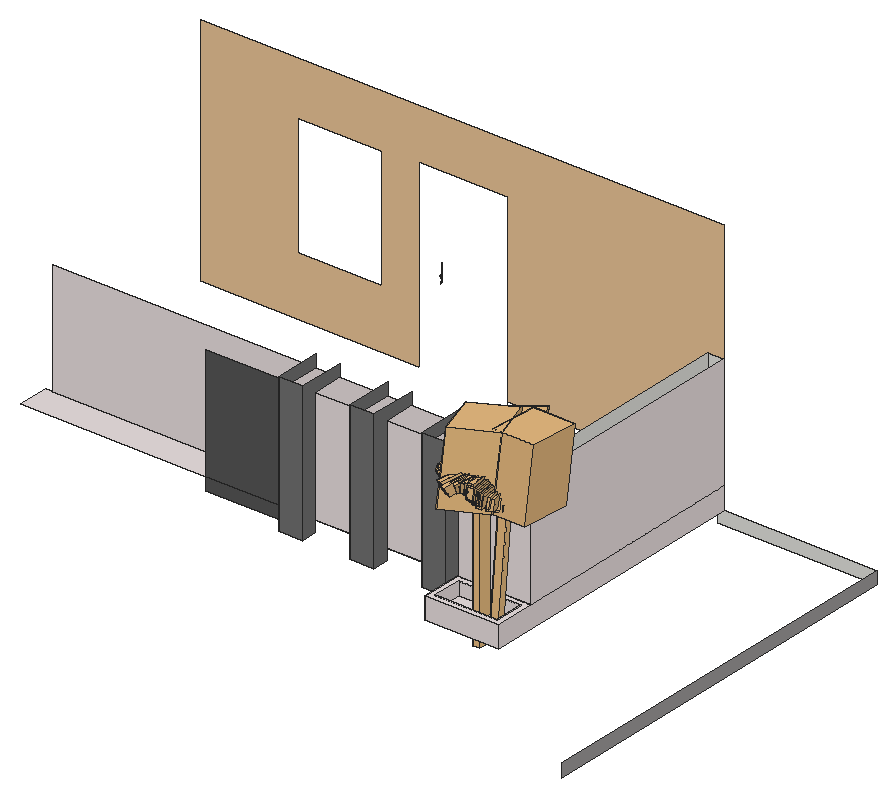
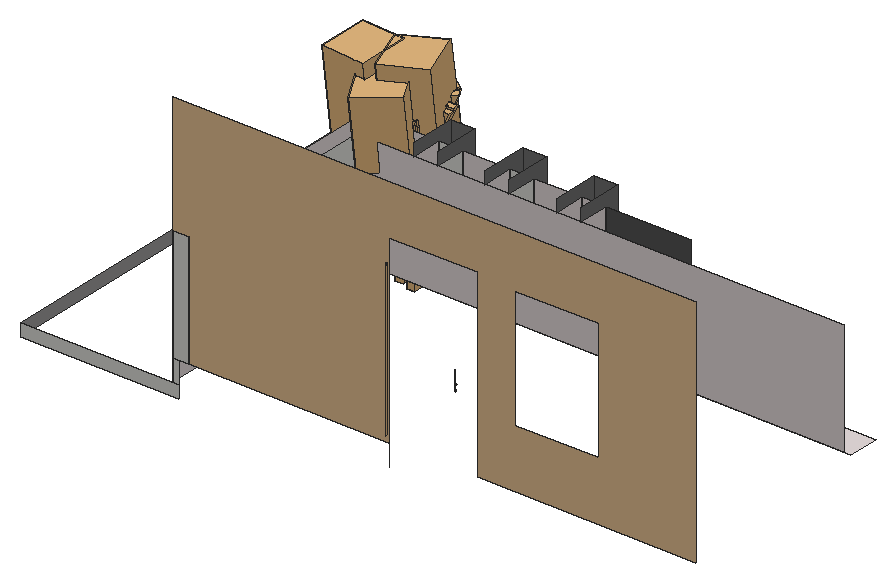
# SketchUp Ruby script. Lengths in inches.
U = 1.inch
M = Sketchup.active_model
def pt(a) = Geom::Point3d.new(a.map { |v| v * U })
def face(e, loops, mat)
  f = e.add_face(loops[0].map { |a| pt(a) })
  loops[1..].each { |l| e.add_face(l.map { |a| pt(a) }).erase! }
  f.material = f.back_material = mat if mat
  f
end
# faces: each face lists its corners as indices into pts; further lists are holes
def faces(e, pts, list, mat = nil) = list.each { |f| face(e, (f[0].is_a?(Array) ? f : [f]).map { |l| l.map { |i| pts[i] } }, mat) }
# xy, xz, yz: faces in a plane at the given z, y or x. An outline is a flat list of corners, or four numbers for a rectangle; further outlines are holes
def ring(l) = l.size == 4 ? [[l[0], l[1]], [l[2], l[1]], [l[2], l[3]], [l[0], l[3]]] : l.each_slice(2).to_a
def flat(e, list, mat, &to3) = list.each { |f| face(e, (f[0].is_a?(Array) ? f : [f]).map { |l| ring(l).map { |u, v| to3.(u, v) } }, mat) }
def xy(e, z, list, mat = nil) = flat(e, list, mat) { |x, y| [x, y, z] }
def xz(e, y, list, mat = nil) = flat(e, list, mat) { |x, z| [x, y, z] }
def yz(e, x, list, mat = nil) = flat(e, list, mat) { |y, z| [x, y, z] }
def lines(e, pts, list) = list.each { |a, b| e.add_line(pt(pts[a]), pt(pts[b])) }
# prism: a flat outline (further loops are holes) pulled along v
def prism(e, loops, v, mat = nil)
  f = face(e, loops, mat); d = Geom::Vector3d.new(v.map { |x| x * U })
  f.pushpull(f.normal.samedirection?(d) ? d.length : -d.length)
end
def box(e, o, s, mat = nil) = prism(e, [[o, [o[0] + s[0], o[1], o[2]], [o[0] + s[0], o[1] + s[1], o[2]], [o[0], o[1] + s[1], o[2]]]], [0, 0, s[2]], mat)
def at(x, y, z, deg = 0) = Geom::Transformation.translation(pt([x, y, z])) * Geom::Transformation.rotation(ORIGIN, Z_AXIS, deg.degrees)
def axes(o, x, y, z) = Geom::Transformation.new([*x, 0, *y, 0, *z, 0, *pt(o).to_a, 1])
def part(name) = M.definitions.add(name)
# library, detail: a bought-in or finely detailed component or shape, given as its bounding box
def library(name, o, s) = part(name).tap { |d| box(d.entities, o, s) }
def detail(e, o, s) = box(e.add_group.entities, o, s)
def put(e, d, t, mat = nil) = e.add_instance(d, t).tap { |i| i.material = mat if mat }
def group(e, t, mat = nil) = e.add_group.tap { |g| g.transformation = t; g.material = mat if mat }.entities
root = M.entities
M.materials.add("AM85_043_leaf").color = [102, 110, 36]
M.materials.add("AM85_043_stem").color = [137, 75, 57]
M.materials.add("Generic\#4").color = [113, 113, 113]
M.materials.add("Generic\#8").color = [235, 197, 151]
M.materials.add("Generic\#9").color = [233, 223, 223]
M.materials.add("Material \#1").color = [140, 140, 140]
M.materials.add("[Color M06]").color = [86, 86, 86]
M.materials.add("[Granite Dark Gray]").color = [158, 155, 155]
c1 = library("3DGeom~9_Defintion",[456.52,-471.89,-18.89],[5.57,1000,5.49])
c2 = library("3DGeom~7_Defintion",[455.56,-471.94,-18.85],[5.55,1000,5.48])
c3 = library("Group\#262",[721.75,-37.78,8.43],[46.9,73.44,671.88])
c4 = library("Group\#253",[26.16,5.88,-22.96],[170.57,196.24,312.95])
c5 = part("Leaf blade")
p = [[83.87,1.9,45.32],[93.74,4.15,37.73],[37.05,-3.5625,61.7],[49.38,-2.58,60.05],[69.4,9.27,54.68],[74.7,9.96,52.16],
  [102.49,6.87,29.18],[110.02,10.09,19.93],[45.83,5.6,61.35],[51.45,6.53,60.35],[91.18,12.19,41.53],[94.56,12.64,38.66],
  [12.82,-5.2,59.53],[24.77,-4.41,61.53],[22.59,0.63,61.46],[34.04,3.3,62.19],[61.47,-1.4,56.68],[73.04,0.08,51.71],
  [109.02,14.97,22.84],[115.89,16.47,11.9375]]
lines(c5.entities,p,[[0,1],[2,3],[4,5],[6,7],[8,9],[10,11],[12,13],[14,15],[16,17],[18,19]])
detail(c5.entities,[1.52,-6.02,0.37],[119.64,24.16,61.82])
c6 = part("Group\#250")
p = [[69.397,177.044,-76.908],[69.056,177.22,-76.772],[69.397,177.397,-76.635],[69.739,177.22,-76.772],[69.397,126.923,-36.489],[68.124,127.405,-35.832],
  [69.397,153.661,-55.129],[70.671,127.405,-35.832],[68.59,154.026,-54.756],[70.205,154.026,-54.756],[69.397,127.887,-35.175],[69.397,154.392,-54.384],
  [69.397,97.5,-21.509],[67.658,98.015,-20.533],[71.137,98.015,-20.533],[69.397,98.53,-19.558],[69.397,66.147,-10.6],[67.192,66.605,-9.289],
  [71.603,66.605,-9.289],[69.397,67.064,-7.977],[69.397,33.682,-4.048],[66.726,33.994,-2.4],[72.069,33.994,-2.4],[69.397,34.304,-0.752],
  [69.397,0.958,-2],[66.26,1.035,-0.035],[69.397,1.112,1.931],[72.535,1.035,-0.035],[69.397,0.956,-2]]
faces(c6.entities,p,[[0,1,2,3]])
faces(c6.entities,p,[[4,5,6],[4,6,7],[8,6,5],[9,7,6],[5,10,11,8],[7,9,11,10],[12,13,4],[12,4,14],
  [5,4,13],[7,14,4],[13,15,10,5],[14,7,10,15],[16,17,12],[16,12,18],[13,12,17],[14,18,12],
  [17,19,15,13],[18,14,15,19],[16,20,17],[16,18,20],[21,17,20],[22,20,18],[21,23,17],[22,18,23],
  [19,17,23],[19,23,18],[20,24,21],[20,22,24],[25,21,24],[25,26,21],[27,24,22],[22,23,27],
  [23,21,26],[28,25,24],[28,27,25],[28,24,27],[26,27,23],[26,25,27]],"AM85_043_stem")
c7 = library("Group\#264",[27.32,5.88,-22.96],[171.91,196.24,312.95])
c8 = library("Group\#274",[721.75,-37.78,8.43],[46.9,73.44,655.53])
xy(root,-6.625,[[458.275,57.753,489.122,72.622]],"Generic\#9")
xy(root,-6,[[408.209,67.75,420.146,75.375],[443.584,67.75,455.521,75.375]])
xy(root,-6,[[372.834,67.75,384.771,75.375]],"Generic\#9")
xy(root,0,[[[455.521,55,491.875,75.375],[458.275,57.753,489.122,72.622]],[238.793,75.375,491.875,75.375,491.875,194.8125,483.886,194.8125,483.886,90.9375,238.793,90.9375]],"Generic\#9")
xy(root,40.593,[[381.979,199.777,381.911,199.796,381.922,199.809],[381.979,199.777,381.922,199.809,381.983,199.793],[381.979,199.777,381.983,199.793,382.051,199.777],[382.051,199.777,381.983,199.793,382.047,199.793],[382.051,199.777,382.047,199.793,382.119,199.796],
  [382.047,199.793,382.108,199.809,382.119,199.796],[381.911,199.796,381.856,199.83,381.872,199.84],[381.911,199.796,381.872,199.84,381.922,199.809],[382.119,199.796,382.108,199.809,382.174,199.83],[382.108,199.809,382.158,199.84,382.174,199.83],
  [381.856,199.83,381.82,199.877,381.84,199.883],[381.856,199.83,381.84,199.883,381.872,199.84],[382.174,199.83,382.158,199.84,382.21,199.877],[382.158,199.84,382.19,199.883,382.21,199.877],[381.82,199.877,381.808,199.93,381.828,199.93],
  [381.82,199.877,381.828,199.93,381.84,199.883],[382.21,199.877,382.19,199.883,382.222,199.93],[382.19,199.883,382.201,199.93,382.222,199.93],[381.808,199.93,381.82,199.984,381.84,199.978],[381.808,199.93,381.84,199.978,381.828,199.93],
  [382.201,199.93,382.19,199.978,382.21,199.984],[382.201,199.93,382.21,199.984,382.222,199.93],[381.84,199.978,381.82,199.984,381.872,200.02],[382.19,199.978,382.158,200.02,382.174,200.03],[382.19,199.978,382.174,200.03,382.21,199.984],
  [381.82,199.984,381.856,200.03,381.872,200.02],[381.872,200.02,381.856,200.03,381.922,200.052],[382.158,200.02,382.108,200.052,382.119,200.065],[382.158,200.02,382.119,200.065,382.174,200.03],[381.856,200.03,381.911,200.065,381.922,200.052],
  [381.922,200.052,381.911,200.065,381.983,200.068],[382.108,200.052,382.047,200.068,382.051,200.084],[382.108,200.052,382.051,200.084,382.119,200.065],[381.911,200.065,381.979,200.084,381.983,200.068],[381.983,200.068,381.979,200.084,382.047,200.068],
  [382.047,200.068,381.979,200.084,382.051,200.084]],"Material \#1")
xy(root,40.61,[[381.979,199.777,381.983,199.793,381.911,199.796],[381.979,199.777,382.047,199.793,381.983,199.793],[381.979,199.777,382.051,199.777,382.047,199.793],[382.051,199.777,382.108,199.809,382.047,199.793],[382.051,199.777,382.119,199.796,382.108,199.809],
  [381.983,199.793,381.922,199.809,381.911,199.796],[381.911,199.796,381.922,199.809,381.856,199.83],[382.119,199.796,382.158,199.84,382.108,199.809],[382.119,199.796,382.174,199.83,382.158,199.84],[381.922,199.809,381.872,199.84,381.856,199.83],
  [381.856,199.83,381.872,199.84,381.82,199.877],[382.174,199.83,382.19,199.883,382.158,199.84],[382.174,199.83,382.21,199.877,382.19,199.883],[381.872,199.84,381.84,199.883,381.82,199.877],[381.82,199.877,381.84,199.883,381.808,199.93],
  [382.21,199.877,382.201,199.93,382.19,199.883],[382.21,199.877,382.222,199.93,382.201,199.93],[381.84,199.883,381.828,199.93,381.808,199.93],[381.808,199.93,381.828,199.93,381.82,199.984],[381.828,199.93,381.84,199.978,381.82,199.984],
  [382.201,199.93,382.222,199.93,382.19,199.978],[382.222,199.93,382.21,199.984,382.19,199.978],[381.84,199.978,381.856,200.03,381.82,199.984],[381.84,199.978,381.872,200.02,381.856,200.03],[382.19,199.978,382.21,199.984,382.158,200.02],
  [382.21,199.984,382.174,200.03,382.158,200.02],[381.872,200.02,381.911,200.065,381.856,200.03],[381.872,200.02,381.922,200.052,381.911,200.065],[382.158,200.02,382.174,200.03,382.108,200.052],[382.174,200.03,382.119,200.065,382.108,200.052],
  [381.922,200.052,381.979,200.084,381.911,200.065],[381.922,200.052,381.983,200.068,381.979,200.084],[382.108,200.052,382.119,200.065,382.047,200.068],[382.119,200.065,382.051,200.084,382.047,200.068],[381.983,200.068,382.051,200.084,381.979,200.084],
  [381.983,200.068,382.047,200.068,382.051,200.084]],"Material \#1")
xy(root,44.421,[[381.979,199.777,381.911,199.796,381.983,199.793],[381.979,199.777,381.983,199.793,382.047,199.793],[381.979,199.777,382.047,199.793,382.051,199.777],[382.051,199.777,382.047,199.793,382.108,199.809],[382.051,199.777,382.108,199.809,382.119,199.796],
  [381.983,199.793,381.911,199.796,381.922,199.809],[381.911,199.796,381.856,199.83,381.922,199.809],[382.119,199.796,382.108,199.809,382.158,199.84],[382.119,199.796,382.158,199.84,382.174,199.83],[381.922,199.809,381.856,199.83,381.872,199.84],
  [381.856,199.83,381.82,199.877,381.872,199.84],[382.174,199.83,382.158,199.84,382.19,199.883],[382.174,199.83,382.19,199.883,382.21,199.877],[381.872,199.84,381.82,199.877,381.84,199.883],[381.82,199.877,381.808,199.93,381.84,199.883],
  [382.21,199.877,382.19,199.883,382.201,199.93],[382.21,199.877,382.201,199.93,382.222,199.93],[381.84,199.883,381.808,199.93,381.828,199.93],[381.808,199.93,381.82,199.984,381.828,199.93],[381.828,199.93,381.82,199.984,381.84,199.978],
  [382.201,199.93,382.19,199.978,382.222,199.93],[382.222,199.93,382.19,199.978,382.21,199.984],[381.84,199.978,381.82,199.984,381.856,200.03],[381.84,199.978,381.856,200.03,381.872,200.02],[382.19,199.978,382.158,200.02,382.21,199.984],
  [382.21,199.984,382.158,200.02,382.174,200.03],[381.872,200.02,381.856,200.03,381.911,200.065],[381.872,200.02,381.911,200.065,381.922,200.052],[382.158,200.02,382.108,200.052,382.174,200.03],[382.174,200.03,382.108,200.052,382.119,200.065],
  [381.922,200.052,381.911,200.065,381.979,200.084],[381.922,200.052,381.979,200.084,381.983,200.068],[382.108,200.052,382.047,200.068,382.119,200.065],[382.119,200.065,382.047,200.068,382.051,200.084],[381.983,200.068,381.979,200.084,382.051,200.084],
  [381.983,200.068,382.051,200.084,382.047,200.068]],"Material \#1")
xy(root,44.438,[[381.979,199.777,381.922,199.809,381.911,199.796],[381.979,199.777,381.983,199.793,381.922,199.809],[381.979,199.777,382.051,199.777,381.983,199.793],[382.051,199.777,382.047,199.793,381.983,199.793],[382.051,199.777,382.119,199.796,382.047,199.793],
  [382.047,199.793,382.119,199.796,382.108,199.809],[381.911,199.796,381.872,199.84,381.856,199.83],[381.911,199.796,381.922,199.809,381.872,199.84],[382.119,199.796,382.174,199.83,382.108,199.809],[382.108,199.809,382.174,199.83,382.158,199.84],
  [381.856,199.83,381.84,199.883,381.82,199.877],[381.856,199.83,381.872,199.84,381.84,199.883],[382.174,199.83,382.21,199.877,382.158,199.84],[382.158,199.84,382.21,199.877,382.19,199.883],[381.82,199.877,381.828,199.93,381.808,199.93],
  [381.82,199.877,381.84,199.883,381.828,199.93],[382.21,199.877,382.222,199.93,382.19,199.883],[382.19,199.883,382.222,199.93,382.201,199.93],[381.808,199.93,381.828,199.93,381.84,199.978],[381.808,199.93,381.84,199.978,381.82,199.984],
  [382.201,199.93,382.21,199.984,382.19,199.978],[382.201,199.93,382.222,199.93,382.21,199.984],[381.84,199.978,381.872,200.02,381.82,199.984],[382.19,199.978,382.174,200.03,382.158,200.02],[382.19,199.978,382.21,199.984,382.174,200.03],
  [381.82,199.984,381.872,200.02,381.856,200.03],[381.872,200.02,381.922,200.052,381.856,200.03],[382.158,200.02,382.119,200.065,382.108,200.052],[382.158,200.02,382.174,200.03,382.119,200.065],[381.856,200.03,381.922,200.052,381.911,200.065],
  [381.922,200.052,381.983,200.068,381.911,200.065],[382.108,200.052,382.051,200.084,382.047,200.068],[382.108,200.052,382.119,200.065,382.051,200.084],[381.911,200.065,381.983,200.068,381.979,200.084],[381.983,200.068,382.047,200.068,381.979,200.084],
  [382.047,200.068,382.051,200.084,381.979,200.084]],"Material \#1")
xz(root,55,[[455.521,-10.875,491.875,0]],"Generic\#9")
xz(root,57.753,[[458.275,-6.625,489.122,0]],"Generic\#9")
xz(root,67.75,[[372.834,-6,384.771,62.5],[408.209,-6,420.146,62.5],[443.584,-6,455.521,62.5]],"Generic\#4")
xz(root,72.622,[[458.275,-6.625,489.122,0]],"Generic\#9")
xz(root,75.375,[[408.209,-6,420.146,0],[443.584,-6,455.521,0],[408.209,0,420.146,56.4375],[443.584,0,455.521,56.4375]])
xz(root,75.375,[[372.834,-6,384.771,0],[372.834,0,384.771,56.4375],[384.771,0,408.209,56.4375],[420.146,0,443.584,56.4375],[455.521,0,491.875,56.4375]],"Generic\#9")
xz(root,75.375,[[330.78,-6,372.834,0],[330.78,0,372.834,56.4375]],"[Color M06]")
xz(root,90.9375,[[242.543,0,483.886,56.4375]],"Generic\#9")
xz(root,194.8125,[[488.6875,-17.3125,567.25,-10.875],[488.6875,-10.875,491.875,0],[483.886,0,491.875,56.4375]])
xz(root,194.8125,[[[232.601,0,340.778,0,340.778,90.9375,384.716,90.9375,384.716,0,483.886,0,483.886,56.4375,491.875,56.4375,491.875,115.8125,232.601,115.8125],[280.759,29.465,322.259,89.402]]],"Generic\#8")
xz(root,199.277,[[347.824,40.059,347.893,40.076,347.86,40.064],[347.824,40.059,347.947,40.12,347.893,40.076],[347.893,40.076,347.947,40.12,347.922,40.095],[347.947,40.12,347.63,40.635,347.668,40.595],[347.947,40.12,347.663,40.549,347.66,40.554],
  [347.947,40.12,347.665,40.543,347.663,40.549],[347.947,40.12,347.666,40.536,347.665,40.543],[347.947,40.12,347.668,40.595,347.714,40.565],[347.947,40.12,347.767,40.546,347.824,40.539],[347.947,40.12,347.824,40.539,347.981,40.221],
  [347.947,40.12,347.977,40.184,347.965,40.15],[347.947,40.12,347.981,40.221,347.977,40.184],[347.981,40.221,347.824,40.539,347.881,40.546],[347.981,40.221,347.881,40.546,347.933,40.565],[347.981,40.221,347.933,40.565,347.979,40.595],
  [347.981,40.221,347.979,40.595,347.981,40.53],[347.981,40.53,347.979,40.595,347.983,40.543],[347.981,40.53,347.983,40.543,347.982,40.537],[347.983,40.543,347.979,40.595,348.018,40.635],[347.983,40.543,347.988,40.555,347.985,40.549],
  [347.983,40.543,348.018,40.635,347.988,40.555],[347.988,40.555,348.018,40.635,348.047,40.682],[347.988,40.555,348.047,40.682,348.103,40.756],[347.988,40.555,348.103,40.756,347.991,40.56],[347.991,40.56,348.103,40.756,347.995,40.565],
  [347.995,40.565,348.048,40.623,348,40.57],[347.995,40.565,348.103,40.756,348.048,40.623],[348,40.57,348.048,40.623,348.026,40.595],[348.048,40.623,348.084,40.685,348.068,40.653],[348.048,40.623,348.103,40.756,348.084,40.685],
  [348.047,40.682,348.066,40.736,348.103,40.756],[348.084,40.685,348.103,40.756,348.096,40.72],[348.066,40.736,348.072,40.794,348.103,40.756],[348.103,40.756,348.044,40.975,348.098,40.861],[348.103,40.756,348.047,40.906,348.044,40.975],
  [348.103,40.756,348.066,40.853,348.047,40.906],[348.103,40.756,348.072,40.794,348.066,40.853],[348.103,40.756,348.098,40.861,348.105,40.794],[348.098,40.861,348.044,40.975,348.077,40.921],[348.047,40.906,348.018,40.954,348.044,40.975],
  [348.018,40.954,347.979,40.993,348.044,40.975],[348.044,40.975,347.824,41.083,347.948,41.054],[348.044,40.975,347.933,41.023,347.824,41.083],[348.044,40.975,347.979,40.993,347.933,41.023],[348.044,40.975,347.948,41.054,348,41.02],
  [347.933,41.023,347.881,41.043,347.824,41.083],[347.881,41.043,347.824,41.049,347.824,41.083],[347.948,41.054,347.824,41.083,347.888,41.076]],"Material \#1")
xz(root,199.308,[[347.824,37.502,347.824,37.514,347.952,37.526],[347.824,37.502,347.952,37.526,347.954,37.514],[347.954,37.514,347.952,37.526,348.072,37.56],[347.954,37.514,348.072,37.56,348.076,37.548],[348.076,37.548,348.072,37.56,348.183,37.614],
  [348.076,37.548,348.183,37.614,348.189,37.603],[348.189,37.603,348.183,37.614,348.282,37.686],[348.189,37.603,348.282,37.686,348.291,37.676],[348.291,37.676,348.282,37.686,348.368,37.774],[348.291,37.676,348.368,37.774,348.378,37.766],
  [347.824,37.7,347.824,37.713,347.865,37.717],[347.824,37.7,347.865,37.717,347.867,37.704],[347.867,37.704,347.865,37.717,347.903,37.728],[347.867,37.704,347.903,37.728,347.908,37.716],[347.908,37.716,347.903,37.728,347.939,37.745],
  [347.908,37.716,347.939,37.745,347.945,37.734],[347.945,37.734,347.939,37.745,347.971,37.768],[347.945,37.734,347.971,37.768,347.979,37.759],[347.979,37.759,347.971,37.768,347.998,37.796],[347.979,37.759,347.998,37.796,348.008,37.788],
  [348.378,37.766,348.368,37.774,348.439,37.876],[348.378,37.766,348.439,37.876,348.45,37.87],[348.008,37.788,347.998,37.796,348.021,37.829],[348.008,37.788,348.021,37.829,348.032,37.823],[348.032,37.823,348.021,37.829,348.038,37.866],
  [348.032,37.823,348.038,37.866,348.049,37.861],[348.049,37.861,348.038,37.866,348.048,37.905],[348.049,37.861,348.048,37.905,348.061,37.903],[348.45,37.87,348.439,37.876,348.491,37.99],[348.45,37.87,348.491,37.99,348.503,37.986],
  [348.061,37.903,348.048,37.905,348.052,37.947],[348.061,37.903,348.052,37.947,348.065,37.947],[348.052,37.947,348.048,37.989,348.065,37.947],[348.065,37.947,348.048,37.989,348.061,37.991],[348.503,37.986,348.491,37.99,348.525,38.113],
  [348.503,37.986,348.525,38.113,348.537,38.111],[348.048,37.989,348.038,38.029,348.061,37.991],[348.061,37.991,348.038,38.029,348.049,38.033],[348.038,38.029,348.021,38.065,348.049,38.033],[348.049,38.033,348.021,38.065,348.032,38.072],
  [348.021,38.065,347.998,38.098,348.032,38.072],[348.032,38.072,347.998,38.098,348.008,38.106],[347.998,38.098,347.971,38.126,348.008,38.106],[348.008,38.106,347.971,38.126,347.979,38.136],[348.537,38.111,348.525,38.113,348.537,38.25],
  [348.537,38.111,348.537,38.25,348.549,38.249],[347.971,38.126,347.939,38.149,347.979,38.136],[347.979,38.136,347.939,38.149,347.945,38.16],[347.939,38.149,347.903,38.167,347.945,38.16],[347.945,38.16,347.903,38.167,347.908,38.179],
  [347.903,38.167,347.865,38.178,347.908,38.179],[347.865,38.178,347.824,38.181,347.867,38.19],[347.865,38.178,347.867,38.19,347.908,38.179],[347.824,38.181,347.824,38.194,347.867,38.19],[348.549,38.249,348.537,38.25,348.537,44.909],
  [348.549,38.249,348.537,44.909,348.537,46.738],[348.549,38.249,348.537,46.738,348.549,46.739]],"Material \#1")
xz(root,199.588,[[347.824,40.059,347.86,40.064,347.893,40.076],[347.754,40.076,347.893,40.076,347.977,40.184],[347.893,40.076,347.922,40.095,347.947,40.12],[347.893,40.076,347.947,40.12,347.977,40.184],[347.947,40.12,347.965,40.15,347.977,40.184],
  [347.977,40.184,347.981,40.221,347.66,40.554],[347.981,40.221,347.824,40.539,347.767,40.546],[347.981,40.221,347.881,40.546,347.824,40.539],[347.981,40.221,347.981,40.53,347.881,40.546],[347.981,40.53,347.983,40.543,347.881,40.546],
  [347.981,40.53,347.982,40.537,347.983,40.543],[347.983,40.543,347.988,40.555,347.881,40.546],[347.983,40.543,347.985,40.549,347.988,40.555],[347.881,40.546,347.988,40.555,347.933,40.565],[347.988,40.555,347.979,40.595,347.933,40.565],
  [347.988,40.555,348.018,40.635,347.979,40.595],[347.988,40.555,347.991,40.56,348.103,40.756],[347.988,40.555,348.103,40.756,348.018,40.635],[347.991,40.56,347.995,40.565,348.103,40.756],[347.995,40.565,348,40.57,348.048,40.623],
  [347.995,40.565,348.048,40.623,348.103,40.756],[348,40.57,348.026,40.595,348.048,40.623],[348.048,40.623,348.068,40.653,348.084,40.685],[348.048,40.623,348.084,40.685,348.103,40.756],[348.018,40.635,348.103,40.756,348.047,40.682],
  [348.047,40.682,348.103,40.756,348.066,40.736],[348.084,40.685,348.096,40.72,348.103,40.756],[348.066,40.736,348.103,40.756,348.072,40.794],[348.103,40.756,348.044,40.975,348.066,40.853],[348.103,40.756,348.098,40.861,348.044,40.975],
  [348.103,40.756,348.066,40.853,348.072,40.794],[348.103,40.756,348.105,40.794,348.098,40.861],[348.066,40.853,348.044,40.975,348.047,40.906],[348.098,40.861,348.077,40.921,348.044,40.975],[348.047,40.906,348.044,40.975,348.018,40.954],
  [348.018,40.954,348.044,40.975,347.979,40.993],[348.044,40.975,347.824,41.083,347.933,41.023],[348.044,40.975,347.948,41.054,347.824,41.083],[348.044,40.975,347.933,41.023,347.979,40.993],[348.044,40.975,348,41.02,347.948,41.054],
  [347.933,41.023,347.824,41.083,347.881,41.043],[347.881,41.043,347.824,41.083,347.824,41.049],[347.948,41.054,347.888,41.076,347.824,41.083]],"Material \#1")
yz(root,347.848,[[199.268,40.718,199.557,40.718,199.557,40.748],[199.268,40.718,199.557,40.748,199.268,40.748]],"Material \#1")
yz(root,347.854,[[199.268,40.837,199.557,40.837,199.557,40.892]],"Material \#1")
yz(root,347.857,[[199.268,40.772,199.557,40.772,199.557,40.796],[199.268,40.772,199.557,40.796,199.268,40.796]],"Material \#1")
yz(root,372.834,[[67.75,-6,67.75,62.5,90.9375,62.5,90.9375,56.4375,75.375,56.4375,75.375,-6]],"Generic\#4")
yz(root,384.771,[[67.75,-6,75.375,-6,75.375,56.4375,90.9375,56.4375,90.9375,62.5,67.75,62.5]],"Generic\#4")
yz(root,408.209,[[67.75,-6,67.75,62.5,90.9375,62.5,90.9375,56.4375,75.375,56.4375,75.375,-6]],"Generic\#4")
yz(root,420.146,[[67.75,-6,75.375,-6,75.375,56.4375,90.9375,56.4375,90.9375,62.5,67.75,62.5]],"Generic\#4")
yz(root,443.584,[[67.75,-6,67.75,62.5,90.9375,62.5,90.9375,56.4375,75.375,56.4375,75.375,-6]],"Generic\#4")
yz(root,455.521,[[67.75,-6,75.375,0],[67.75,0,75.375,0,75.375,56.4375,90.9375,56.4375,90.9375,62.5,67.75,62.5]],"Generic\#4")
yz(root,455.521,[[55,-10.875,55,0,67.75,0,67.75,-6,75.375,-6,75.375,-10.875]],"Generic\#9")
yz(root,458.275,[[57.753,-6.625,72.622,0]],"Generic\#9")
yz(root,483.886,[[90.9375,0,194.8125,56.4375]])
yz(root,489.122,[[57.753,-6.625,72.622,0]],"Generic\#9")
yz(root,491.875,[[55,-10.875,194.8125,0],[75.375,0,194.8125,56.4375]],"Generic\#9")
yz(root,567.25,[[0,-17.3125,194.8125,-10.875]],"[Granite Dark Gray]")
p = [[347.839,199.268,40.654],[347.836,199.557,40.65],[347.842,199.557,40.658],[347.836,199.557,40.65],[347.839,199.268,40.654],[347.848,199.268,40.624],
  [347.848,199.268,40.624],[347.848,199.557,40.624],[347.836,199.557,40.65],[347.839,199.268,40.682],[347.842,199.557,40.678],[347.836,199.557,40.686],
  [347.839,199.268,40.654],[347.842,199.557,40.658],[347.842,199.557,40.678],[347.839,199.268,40.682],[347.839,199.268,40.682],[347.836,199.557,40.686],
  [347.848,199.557,40.718],[347.848,199.557,40.718],[347.848,199.268,40.718],[347.839,199.268,40.682],[347.848,199.268,40.748],[347.848,199.557,40.748],
  [347.857,199.557,40.772],[347.857,199.557,40.772],[347.857,199.268,40.772],[347.848,199.268,40.748],[347.848,199.268,40.82],[347.848,199.557,40.82],
  [347.854,199.557,40.837],[347.848,199.557,40.82],[347.848,199.268,40.82],[347.857,199.268,40.796],[347.854,199.557,40.837],[347.854,199.268,40.837],
  [347.848,199.268,40.82],[347.857,199.268,40.796],[347.857,199.557,40.796],[347.848,199.557,40.82],[347.854,199.557,40.892],[347.851,199.268,40.902],
  [347.854,199.268,40.837],[347.851,199.268,40.902],[347.854,199.557,40.909],[347.854,199.557,40.964],[347.854,199.557,40.964],[347.854,199.268,40.964],
  [347.851,199.268,40.902],[384.716,194.8125,0],[384.716,194.8125,-10.875]]
faces(root,p,[[0,1,2],[3,4,5],[6,7,8],[9,10,11],[12,13,14],[14,15,12],[16,17,18],[19,20,21],
  [22,23,24],[25,26,27],[28,29,30],[31,32,33],[34,35,36],[37,38,39],[40,41,42],[43,44,45],
  [46,47,48]],"Material \#1")
lines(root,p,[[49,50]])
put(root,c1,axes([347.82,200.83,42.49],[0.07444,0,0],[0,0,0.07633],[0,0.05589,0]),"Material \#1")
put(root,c2,axes([347.82,200.83,42.49],[0.0746,0,0],[0,0,0.07649],[0,0.05601,0]),"Material \#1")
put(root,c3,axes([417.33,65.83,-20.57],[0.07708,0,0],[0,0.07708,0],[0,0,0.14182]))
put(root,c4,axes([488.96,54.34,48.94],[-0.04493,0.13029,-0.00598],[-0.09954,-0.05218,-0.0001],[0.01355,0.00122,0.1207]))
g1 = group(root,at(491.99,58.79,47.98),"AM85_043_leaf")
put(g1,c5,axes([-9.23,-11.07,8.82],[-0.01235,0.13451,0.00409],[-0.13076,-0.00062,-0.00166],[0.01365,-0.02038,0.08907]))
put(g1,c5,axes([-7.38,-11.68,9.59],[-0.02475,0.14517,-0.00613],[-0.12897,-0.01477,-0.00217],[0.00998,0.0009,0.08893]))
put(g1,c5,axes([-24.98,13.875,6.9],[0.11613,-0.04123,0.00406],[-0.03903,-0.14246,0.00467],[0.00998,0.0009,0.08893]))
put(g1,c5,axes([-1.1875,-0.79,0.09],[-0.04662,0.10052,-0.00487],[-0.10816,-0.07548,0.00062],[0.00998,0.0009,0.08893]))
put(g1,c5,axes([-24.41,-9.45,11.04],[0.09363,0.08954,0.00274],[-0.08871,0.13371,-0.0069],[-0.01617,-0.02372,0.06395]))
put(g1,c5,axes([-4.21,-10.02,5.46],[-0.0278,0.16312,-0.00689],[-0.12897,-0.01477,-0.00217],[0.00998,0.0009,0.08893]))
put(g1,c5,axes([-1.64,-6.25,2.61],[-0.04278,0.14054,-0.00633],[-0.11629,-0.05416,-0.00038],[0.00998,0.0009,0.08893]))
put(g1,c5,axes([-1.3,-0.96,0.92],[-0.04662,0.10052,-0.00487],[-0.10816,-0.07548,0.00062],[0.00998,0.0009,0.08893]))
put(g1,c5,axes([-3.77,-10.4375,4.63],[-0.0278,0.16312,-0.00689],[-0.12897,-0.01477,-0.00217],[0.00998,0.0009,0.08893]))
put(g1,c5,axes([-24.38,10.18,7.57],[0.09883,-0.02333,0.01254],[-0.02873,-0.14547,0.0061],[-0.00522,0.00642,0.08764]))
put(g1,c5,axes([-11.09,-11.12,8.99],[-0.00248,0.12905,0.00666],[-0.13166,0.01357,-0.00188],[0.0128,-0.02617,0.08882]))
put(g1,c5,axes([-4.39,-11.26,6.22],[-0.0278,0.16312,-0.00689],[-0.12897,-0.01477,-0.00217],[0.00998,0.0009,0.08893]))
put(g1,c5,axes([-28.79,0.21,7.66],[0.11531,0.04246,0.02918],[0.03432,-0.13956,-0.00186],[-0.02521,-0.02673,0.08422]))
put(g1,c5,axes([-28.54,2.5625,6.88],[0.11652,0.0256,0.034],[0.01721,-0.14582,0.00621],[-0.03519,-0.00873,0.08218]))
put(g1,c5,axes([-23.7,15.89,4.66],[0.11613,-0.04123,0.00406],[-0.03903,-0.14246,0.00467],[0.00998,0.0009,0.08893]))
put(g1,c5,axes([-23.02,16.59,4.64],[0.11613,-0.04123,0.00406],[-0.03903,-0.14246,0.00467],[0.00998,0.0009,0.08893]))
put(g1,c5,axes([-24.27,15.68,5.57],[0.11613,-0.04123,0.00406],[-0.03903,-0.14246,0.00467],[0.00998,0.0009,0.08893]))
put(g1,c5,axes([-4.66,-11.6,6.76],[-0.0278,0.16312,-0.00689],[-0.12897,-0.01477,-0.00217],[0.00998,0.0009,0.08893]))
put(g1,c5,axes([-16.37,-14.45,7.9],[0.03446,0.1421,0.02776],[-0.12772,0.05994,-0.00481],[-0.0025,-0.05513,0.08466]))
put(g1,c5,axes([-25.78,-6.65,11.37],[0.0877,0.09795,0.00229],[0.08092,-0.10711,0.006],[-0.01617,-0.02372,0.06395]))
put(g1,c5,axes([-19.63,19.02,1.15],[0.09598,-0.05646,0.00422],[-0.06578,-0.12586,0.00346],[0.00998,0.0009,0.08893]))
put(g1,c5,axes([-15.72,19.24,-0.27],[0.06517,-0.05819,0.00363],[-0.07999,-0.11548,0.00276],[0.00998,0.0009,0.08893]))
put(g1,c5,axes([-23.07,16.71,3.07],[0.11613,-0.04123,0.00406],[-0.03903,-0.14246,0.00467],[0.00998,0.0009,0.08893]))
put(g1,c5,axes([-24.6,13.3,7.95],[0.10336,-0.0367,0.00361],[-0.03903,-0.14246,0.00467],[0.00998,0.0009,0.08893]))
put(g1,c5,axes([-24.75,14.35,6.37],[0.11613,-0.04123,0.00406],[-0.03903,-0.14246,0.00467],[0.00998,0.0009,0.08893]))
put(g1,c5,axes([-5.67,-12.26,7.875],[-0.0278,0.16312,-0.00689],[-0.12897,-0.01477,-0.00217],[0.00998,0.0009,0.08893]))
put(g1,c5,axes([-6.45,-13.19,8.97],[-0.0278,0.16312,-0.00689],[-0.12897,-0.01477,-0.00217],[0.00998,0.0009,0.08893]))
put(g1,c5,axes([-18.4,-14.27,8.54],[0.04888,0.13676,0.02412],[-0.12169,0.08191,-0.01373],[-0.01758,-0.03757,0.0848]))
put(g1,c5,axes([-6.0625,-12.73,8.43],[-0.0278,0.16312,-0.00689],[-0.12897,-0.01477,-0.00217],[0.00998,0.0009,0.08893]))
put(g1,c5,axes([-5.28,-11.79,7.33],[-0.0278,0.16312,-0.00689],[-0.12897,-0.01477,-0.00217],[0.00998,0.0009,0.08893]))
put(g1,c5,axes([-24.17,12.4375,7.99],[0.10336,-0.0367,0.00361],[-0.03903,-0.14246,0.00467],[0.00998,0.0009,0.08893]))
put(g1,c5,axes([-15.21,-11.37,8.56],[0.02711,0.12247,0.01622],[-0.12583,0.04906,0.01118],[0.02464,-0.05146,0.08634]))
put(g1,c5,axes([-24.8125,8.09,7.86],[0.09705,-0.01226,0.01423],[-0.01827,-0.1474,0.00674],[-0.00978,0.00588,0.0871]))
put(g1,c5,axes([-2.86,-7.27,3.6875],[-0.03457,0.14397,-0.00629],[-0.11899,-0.04423,-0.00082],[0.00998,0.0009,0.08893]))
put(g1,c5,axes([-24.38,15.29,6.55],[0.11613,-0.04123,0.00406],[-0.03903,-0.14246,0.00467],[0.00998,0.0009,0.08893]))
put(g1,c5,axes([-25.92,3.58,7.65],[0.09924,0.02007,0.02171],[0.01072,-0.1448,0.02156],[-0.02645,0.02107,0.08245]))
put(g1,c5,axes([-20.57,17.61,2.25],[0.10033,-0.04754,0.00397],[-0.05893,-0.12949,0.00375],[0.00998,0.0009,0.08893]))
put(g1,c6,axes([-0.98,-0.4,-0.05],[-0.1136,0.16128,-0.00864],[-0.00302,-0.01193,0.08201],[0.09459,0.09727,0.01354]))
g2 = group(root,at(480.82,63,43.49))
put(g2,c5,axes([-5.18,4.84,5.66],[0.04784,0.02128,0.00682],[-0.0261,0.06849,-0.00244],[-0.00026,-0.00359,0.06117]))
put(g2,c5,axes([-5,3.85,6.19],[0.04883,0.02828,-0.00005],[-0.03104,0.06599,-0.00321],[0.00693,0.00063,0.06169]))
put(g2,c5,axes([0.89,15.68,4.9375],[0.00777,-0.06517,0.00268],[-0.06047,0.00541,-0.00149],[0.00693,0.00063,0.06169]))
put(g2,c5,axes([-0.23,1.16,0.01],[0.02796,0.03502,-0.00076],[-0.04939,0.04868,-0.00293],[0.00693,0.00063,0.06169]))
put(g2,c5,axes([-7.46,13.13,7.1],[0.05193,-0.03932,0.00554],[0.03191,0.06058,-0.00156],[-0.00869,0.01008,0.04339]))
put(g2,c5,axes([-3.98,2.1,3.41],[0.05486,0.03177,-0.00006],[-0.03104,0.06599,-0.00321],[0.00693,0.00063,0.06169]))
put(g2,c5,axes([-2.22,0.97,1.58],[0.04354,0.03723,-0.00051],[-0.04311,0.05519,-0.00305],[0.00693,0.00063,0.06169]))
put(g2,c5,axes([-0.27,1.25,0.58],[0.02796,0.03502,-0.00076],[-0.04939,0.04868,-0.00293],[0.00693,0.00063,0.06169]))
put(g2,c5,axes([-4.09,1.77,2.83],[0.05486,0.03177,-0.00006],[-0.03104,0.06599,-0.00321],[0.00693,0.00063,0.06169]))
put(g2,c5,axes([-0.33,15.01,5.3],[0.01146,-0.0536,0.00893],[-0.05948,-0.00023,-0.00049],[0.00591,0.00912,0.06081]))
put(g2,c5,axes([-5.5625,5.82,5.76],[0.04788,0.01567,0.00852],[-0.02101,0.07048,-0.00217],[-0.0026,-0.00378,0.06081]))
put(g2,c5,axes([-4.43,2.11,3.9],[0.05486,0.03177,-0.00006],[-0.03104,0.06599,-0.00321],[0.00693,0.00063,0.06169]))
put(g2,c5,axes([-4.9,16.25,5.01],[0.04005,-0.05407,0.02262],[-0.04527,-0.03321,-0.00522],[-0.01054,0.01582,0.05724]))
put(g2,c5,axes([-4.02,16.32,4.55],[0.03427,-0.05621,0.02545],[-0.05055,-0.02438,0.00002],[-0.00592,0.02286,0.05628]))
put(g2,c5,axes([1.78,15.07,3.46],[0.00777,-0.06517,0.00268],[-0.06047,0.00541,-0.00149],[0.00693,0.00063,0.06169]))
put(g2,c5,axes([2.18,14.79,3.48],[0.00777,-0.06517,0.00268],[-0.06047,0.00541,-0.00149],[0.00693,0.00063,0.06169]))
put(g2,c5,axes([1.64,15.41,4.08],[0.00777,-0.06517,0.00268],[-0.06047,0.00541,-0.00149],[0.00693,0.00063,0.06169]))
put(g2,c5,axes([-4.59,2.25,4.27],[0.05486,0.03177,-0.00006],[-0.03104,0.06599,-0.00321],[0.00693,0.00063,0.06169]))
put(g2,c5,axes([-7.9,8.16,4.85],[0.06112,-0.00094,0.02389],[-0.00313,0.07323,-0.00274],[-0.01661,0.00085,0.0569]))
put(g2,c5,axes([-6.67,14.17,7.4],[0.05387,-0.03533,0.00542],[-0.02359,-0.05367,0.00167],[-0.00869,0.01008,0.04339]))
put(g2,c5,axes([3.57,13.05,1.17],[-0.00187,-0.05622,0.00213],[-0.05963,0.02117,-0.00208],[0.00693,0.00063,0.06169]))
put(g2,c5,axes([4.34,10.93,0.23],[-0.00862,-0.04027,0.00137],[-0.05861,0.02971,-0.00239],[0.00693,0.00063,0.06169]))
put(g2,c5,axes([2.125,14.73,2.39],[0.00777,-0.06517,0.00268],[-0.06047,0.00541,-0.00149],[0.00693,0.00063,0.06169]))
put(g2,c5,axes([0.8125,15.48,5.65],[0.00691,-0.058,0.00239],[-0.06047,0.00541,-0.00149],[0.00693,0.00063,0.06169]))
put(g2,c5,axes([1.09,15.58,4.59],[0.00777,-0.06517,0.00268],[-0.06047,0.00541,-0.00149],[0.00693,0.00063,0.06169]))
put(g2,c5,axes([-4.97,2.78,5],[0.05486,0.03177,-0.00006],[-0.03104,0.06599,-0.00321],[0.00693,0.00063,0.06169]))
put(g2,c5,axes([-5.41,3.16,5.73],[0.05486,0.03177,-0.00006],[-0.03104,0.06599,-0.00321],[0.00693,0.00063,0.06169]))
put(g2,c5,axes([-8.2,9.29,5.28],[0.06179,-0.00933,0.02135],[0.00578,0.07186,-0.00819],[-0.01304,0.01068,0.05739]))
put(g2,c5,axes([-5.2,2.97,5.37],[0.05486,0.03177,-0.00006],[-0.03104,0.06599,-0.00321],[0.00693,0.00063,0.06169]))
put(g2,c5,axes([-4.75,2.59,4.65],[0.05486,0.03177,-0.00006],[-0.03104,0.06599,-0.00321],[0.00693,0.00063,0.06169]))
put(g2,c5,axes([0.58,15.17,5.66],[0.00691,-0.058,0.00239],[-0.06047,0.00541,-0.00149],[0.00693,0.00063,0.06169]))
put(g2,c5,axes([-6.49,7.93,5.41],[0.05176,0.00004,0.01523],[-0.00597,0.0721,0.00801],[-0.00981,-0.01289,0.05844]))
put(g2,c5,axes([-1.17,15.03,5.43],[0.01531,-0.05136,0.01042],[-0.05811,-0.00589,-0.00001],[0.00479,0.01142,0.06038]))
put(g2,c5,axes([-2.78,1.57,2.29],[0.04644,0.03329,-0.0003],[-0.03996,0.05765,-0.00307],[0.00693,0.00063,0.06169]))
put(g2,c5,axes([1.52,15.49,4.75],[0.00777,-0.06517,0.00268],[-0.06047,0.00541,-0.00149],[0.00693,0.00063,0.06169]))
put(g2,c5,axes([-3.08,15.11,5.14],[0.02816,-0.04854,0.0166],[-0.05065,-0.01987,0.01061],[0.00691,0.02152,0.05747]))
put(g2,c5,axes([2.91,13.46,1.875],[0.0023,-0.05756,0.00227],[-0.05962,0.0172,-0.00193],[0.00693,0.00063,0.06169]))
put(g2,c6,axes([-0.05,1.08,-0.08],[0.03717,0.07651,-0.00216],[-0.00077,0.00562,0.05638],[0.05556,-0.03829,0.01326]))
put(root,c7,axes([472.61,58.85,46.69],[0.0969,0.08105,-0.00107],[-0.06023,0.10764,-0.00543],[0.01165,0.00105,0.1038]))
put(root,c8,axes([481.55,111.45,-19.56],[-0.002,-0.05855,0.00173],[0.05849,-0.00203,-0.00181],[0.00589,0.00229,0.10018]))
put(root,c4,axes([482.8,85.89,47.59],[-0.00486,-0.14197,0.00538],[0.10774,-0.00353,0.00242],[0.01355,0.00122,0.1207]))
